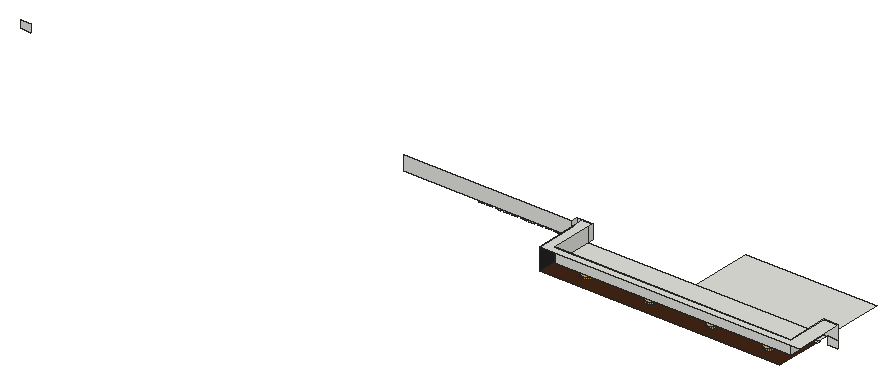
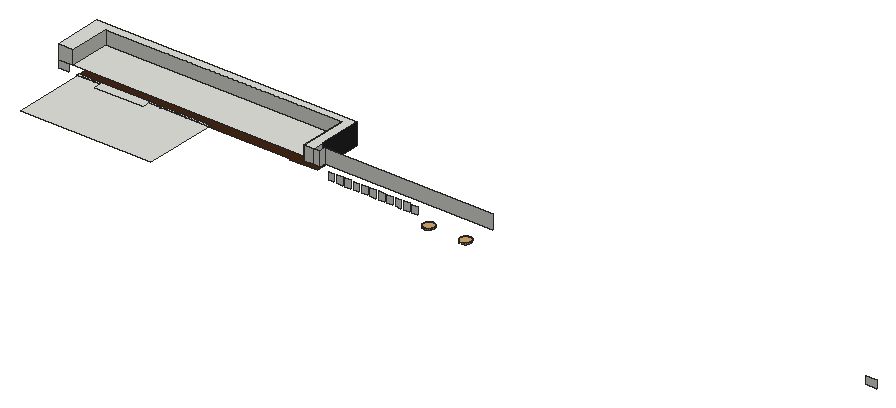
# SketchUp Ruby script. Lengths in inches.
U = 1.inch
M = Sketchup.active_model
def pt(a) = Geom::Point3d.new(a.map { |v| v * U })
def face(e, loops, mat)
  f = e.add_face(loops[0].map { |a| pt(a) })
  loops[1..].each { |l| e.add_face(l.map { |a| pt(a) }).erase! }
  f.material = f.back_material = mat if mat
  f
end
# faces: each face lists its corners as indices into pts; further lists are holes
def faces(e, pts, list, mat = nil) = list.each { |f| face(e, (f[0].is_a?(Array) ? f : [f]).map { |l| l.map { |i| pts[i] } }, mat) }
# xy, xz, yz: faces in a plane at the given z, y or x. An outline is a flat list of corners, or four numbers for a rectangle; further outlines are holes
def ring(l) = l.size == 4 ? [[l[0], l[1]], [l[2], l[1]], [l[2], l[3]], [l[0], l[3]]] : l.each_slice(2).to_a
def flat(e, list, mat, &to3) = list.each { |f| face(e, (f[0].is_a?(Array) ? f : [f]).map { |l| ring(l).map { |u, v| to3.(u, v) } }, mat) }
def xy(e, z, list, mat = nil) = flat(e, list, mat) { |x, y| [x, y, z] }
def xz(e, y, list, mat = nil) = flat(e, list, mat) { |x, z| [x, y, z] }
def yz(e, x, list, mat = nil) = flat(e, list, mat) { |y, z| [x, y, z] }
def lines(e, pts, list) = list.each { |a, b| e.add_line(pt(pts[a]), pt(pts[b])) }
# prism: a flat outline (further loops are holes) pulled along v
def prism(e, loops, v, mat = nil)
  f = face(e, loops, mat); d = Geom::Vector3d.new(v.map { |x| x * U })
  f.pushpull(f.normal.samedirection?(d) ? d.length : -d.length)
end
def box(e, o, s, mat = nil) = prism(e, [[o, [o[0] + s[0], o[1], o[2]], [o[0] + s[0], o[1] + s[1], o[2]], [o[0], o[1] + s[1], o[2]]]], [0, 0, s[2]], mat)
def at(x, y, z, deg = 0) = Geom::Transformation.translation(pt([x, y, z])) * Geom::Transformation.rotation(ORIGIN, Z_AXIS, deg.degrees)
def axes(o, x, y, z) = Geom::Transformation.new([*x, 0, *y, 0, *z, 0, *pt(o).to_a, 1])
def part(name) = M.definitions.add(name)
# library, detail: a bought-in or finely detailed component or shape, given as its bounding box
def library(name, o, s) = part(name).tap { |d| box(d.entities, o, s) }
def detail(e, o, s) = box(e.add_group.entities, o, s)
def put(e, d, t, mat = nil) = e.add_instance(d, t).tap { |i| i.material = mat if mat }
def group(e, t, mat = nil) = e.add_group.tap { |g| g.transformation = t; g.material = mat if mat }.entities
root = M.entities
M.materials.add("[Field Square Tile]").color = [211, 167, 108]
M.materials.add("[Granite Dark Gray]").color = [38, 37, 37]
M.materials.add("[Wood Veneer 01]").color = [66, 38, 20]
xy(root,380.5,[[1413.21,2343.96,1418.63,2346.71],[1418.63,2343.96,1419.83,2346.71],[1419.83,2343.96,1425.26,2346.71],[1425.26,2343.96,1426.46,2346.71],[1426.46,2343.96,1431.88,2346.71],
  [1431.88,2343.96,1433.08,2346.71],[1433.08,2343.96,1438.51,2346.71],[1438.51,2343.96,1439.71,2346.71],[1439.71,2343.96,1445.13,2346.71],[1445.13,2343.96,1446.33,2346.71],
  [1446.33,2343.96,1451.76,2346.71],[1451.76,2343.96,1452.96,2346.71],[1452.96,2343.96,1458.38,2346.71],[1458.38,2343.96,1459.58,2346.71],[1459.58,2343.96,1465.01,2346.71],
  [1465.01,2343.96,1466.21,2346.71],[1466.21,2343.96,1471.63,2346.71],[1471.63,2343.96,1472.83,2346.71],[1472.83,2343.96,1478.26,2346.71],[1478.26,2343.96,1531.81,2354.27],
  [1531.81,2343.96,1537.23,2346.71],[1537.23,2343.96,1538.43,2346.71],[1538.43,2343.96,1543.86,2346.71],[1543.86,2343.96,1545.06,2346.71],[1545.06,2343.96,1550.48,2346.71],
  [1550.48,2343.96,1551.31,2346.71],[1551.31,2343.96,1555.29,2346.71],[1555.29,2343.96,1556.73,2346.71],[1413.21,2346.71,1413.21,2425.46,1555.29,2425.46,1555.29,2346.71,1531.81,2346.71,1531.81,2354.27,1478.26,2354.27,1478.26,2346.71]])
xy(root,380.5,[[[1293.73,2294.125,1293.73,2347.9,1323.53,2347.9,1323.53,2346.71,1413.21,2346.71,1413.21,2343.96,1555.29,2343.96,1555.29,2294.125],[1529.08,2306.32,1530.64,2306.53,1532.08,2307.13,1533.33,2308.08,1534.28,2309.32,1534.88,2310.77,1535.08,2312.32,1534.88,2313.88,1534.28,2315.32,1533.33,2316.57,1532.08,2317.52,1530.64,2318.12,1529.08,2318.32,1527.53,2318.12,1526.08,2317.52,1524.84,2316.57,1523.89,2315.32,1523.29,2313.88,1523.08,2312.32,1523.29,2310.77,1523.89,2309.32,1524.84,2308.08,1526.08,2307.13,1527.53,2306.53],[1400.43,2306.32,1401.98,2306.53,1403.43,2307.13,1404.67,2308.08,1405.63,2309.32,1406.23,2310.77,1406.43,2312.32,1406.23,2313.88,1405.63,2315.32,1404.67,2316.57,1403.43,2317.52,1401.98,2318.12,1400.43,2318.32,1398.88,2318.12,1397.43,2317.52,1396.1875,2316.57,1395.24,2315.32,1394.64,2313.88,1394.43,2312.32,1394.64,2310.77,1395.24,2309.32,1396.1875,2308.08,1397.43,2307.13,1398.88,2306.53],[1330.97,2306.32,1332.52,2306.53,1333.97,2307.13,1335.21,2308.08,1336.16,2309.32,1336.76,2310.77,1336.97,2312.32,1336.76,2313.88,1336.16,2315.32,1335.21,2316.57,1333.97,2317.52,1332.52,2318.12,1330.97,2318.32,1329.42,2318.12,1327.97,2317.52,1326.73,2316.57,1325.77,2315.32,1325.17,2313.88,1324.97,2312.32,1325.17,2310.77,1325.77,2309.32,1326.73,2308.08,1327.97,2307.13,1329.42,2306.53],[1467.71,2306.32,1469.26,2306.53,1470.71,2307.13,1471.95,2308.08,1472.91,2309.32,1473.51,2310.77,1473.71,2312.32,1473.51,2313.88,1472.91,2315.32,1471.95,2316.57,1470.71,2317.52,1469.26,2318.12,1467.71,2318.32,1466.16,2318.12,1464.71,2317.52,1463.47,2316.57,1462.51,2315.32,1461.91,2313.88,1461.71,2312.32,1461.91,2310.77,1462.51,2309.32,1463.47,2308.08,1464.71,2307.13,1466.16,2306.53]]],"[Wood Veneer 01]")
xy(root,381.8125,[[1330.97,2306.32,1329.42,2306.53,1327.97,2307.13,1326.73,2308.08,1325.77,2309.32,1325.17,2310.77,1324.97,2312.32,1325.17,2313.88,1325.77,2315.32,1326.73,2316.57,1327.97,2317.52,1329.42,2318.12,1330.97,2318.32,1332.52,2318.12,1333.97,2317.52,1335.21,2316.57,1336.16,2315.32,1336.76,2313.88,1336.97,2312.32,1336.76,2310.77,1336.16,2309.32,1335.21,2308.08,1333.97,2307.13,1332.52,2306.53],[1400.43,2306.32,1398.88,2306.53,1397.43,2307.13,1396.1875,2308.08,1395.24,2309.32,1394.64,2310.77,1394.43,2312.32,1394.64,2313.88,1395.24,2315.32,1396.1875,2316.57,1397.43,2317.52,1398.88,2318.12,1400.43,2318.32,1401.98,2318.12,1403.43,2317.52,1404.67,2316.57,1405.63,2315.32,1406.23,2313.88,1406.43,2312.32,1406.23,2310.77,1405.63,2309.32,1404.67,2308.08,1403.43,2307.13,1401.98,2306.53],[1467.71,2306.32,1466.16,2306.53,1464.71,2307.13,1463.47,2308.08,1462.51,2309.32,1461.91,2310.77,1461.71,2312.32,1461.91,2313.88,1462.51,2315.32,1463.47,2316.57,1464.71,2317.52,1466.16,2318.12,1467.71,2318.32,1469.26,2318.12,1470.71,2317.52,1471.95,2316.57,1472.91,2315.32,1473.51,2313.88,1473.71,2312.32,1473.51,2310.77,1472.91,2309.32,1471.95,2308.08,1470.71,2307.13,1469.26,2306.53],[1529.08,2306.32,1527.53,2306.53,1526.08,2307.13,1524.84,2308.08,1523.89,2309.32,1523.29,2310.77,1523.08,2312.32,1523.29,2313.88,1523.89,2315.32,1524.84,2316.57,1526.08,2317.52,1527.53,2318.12,1529.08,2318.32,1530.64,2318.12,1532.08,2317.52,1533.33,2316.57,1534.28,2315.32,1534.88,2313.88,1535.08,2312.32,1534.88,2310.77,1534.28,2309.32,1533.33,2308.08,1532.08,2307.13,1530.64,2306.53]],"[Field Square Tile]")
xy(root,381.875,[[1119.58,2359.13,1118.02,2359.16,1116.51,2359.6,1115.17,2360.41,1114.09,2361.54,1113.33,2362.91,1112.96,2364.4375,1112.99,2366,1113.43,2367.51,1114.24,2368.85,1115.37,2369.93,1116.74,2370.69,1118.26,2371.06,1119.83,2371.03,1121.33,2370.59,1122.67,2369.78,1123.76,2368.65,1124.51,2367.28,1124.89,2365.75,1124.85,2364.1875,1124.42,2362.68,1123.61,2361.34,1122.48,2360.26,1121.1,2359.51],[1159.33,2359.13,1157.77,2359.16,1156.26,2359.6,1154.92,2360.41,1153.84,2361.54,1153.08,2362.91,1152.71,2364.4375,1152.74,2366,1153.18,2367.51,1153.99,2368.85,1155.12,2369.93,1156.49,2370.69,1158.01,2371.06,1159.58,2371.03,1161.08,2370.59,1162.42,2369.78,1163.51,2368.65,1164.26,2367.28,1164.64,2365.75,1164.6,2364.1875,1164.17,2362.68,1163.36,2361.34,1162.23,2360.26,1160.85,2359.51]],"[Field Square Tile]")
xy(root,388.625,[[1304.4375,2301.68,1560.93,2346.71]])
xy(root,403.8125,[[1293.73,2294.125,1576.91,2294.125,1576.91,2346.71,1560.93,2346.71,1560.93,2301.68,1304.4375,2301.68,1304.4375,2353.05,1293.73,2353.05]])
xz(root,2301.68,[[1304.4375,388.625,1560.93,403.8125]])
xz(root,2346.49,[[1104.06,388.625,1287.38,403.8125]])
xz(root,2346.71,[[686.35,380.5,698.16,388.625],[1565.1,380.5,1576.91,388.625],[1560.93,388.625,1576.91,403.8125]])
xz(root,2353.05,[[1287.38,388.625,1293.73,403.8125],[1293.73,388.625,1304.4375,403.8125]])
xz(root,2355.06,[[1178.68,380.5,1184.93,388.625],[1187.81,380.5,1194.06,388.625],[1196.93,380.5,1203.18,388.625],[1206.06,380.5,1212.31,388.625],[1215.18,380.5,1221.43,388.625],
  [1224.31,380.5,1230.56,388.625],[1233.43,380.5,1239.68,388.625],[1242.56,380.5,1248.81,388.625],[1251.68,380.5,1257.93,388.625],[1260.81,380.5,1267.06,388.625],
  [1269.93,380.5,1276.18,388.625]])
yz(root,1287.38,[[2346.49,388.625,2353.05,403.8125]])
yz(root,1293.73,[[2294.125,380.5,2340.15,403.8125]],"[Granite Dark Gray]")
yz(root,1304.4375,[[2301.68,388.625,2346.71,403.8125],[2346.71,388.625,2353.05,403.8125]])
yz(root,1560.93,[[2301.68,388.625,2346.71,403.8125]])
p = [[1330.97,2306.32,380.5],[1329.42,2306.53,380.5],[1329.42,2306.53,381.8125],[1330.97,2306.32,381.8125],[1332.52,2306.53,380.5],[1332.52,2306.53,381.8125],
  [1400.43,2306.32,380.5],[1398.88,2306.53,380.5],[1398.88,2306.53,381.8125],[1400.43,2306.32,381.8125],[1401.98,2306.53,380.5],[1401.98,2306.53,381.8125],
  [1467.71,2306.32,380.5],[1466.16,2306.53,380.5],[1466.16,2306.53,381.8125],[1467.71,2306.32,381.8125],[1469.26,2306.53,380.5],[1469.26,2306.53,381.8125],
  [1529.08,2306.32,380.5],[1527.53,2306.53,380.5],[1527.53,2306.53,381.8125],[1529.08,2306.32,381.8125],[1530.64,2306.53,380.5],[1530.64,2306.53,381.8125],
  [1327.97,2307.13,380.5],[1327.97,2307.13,381.8125],[1333.97,2307.13,380.5],[1333.97,2307.13,381.8125],[1397.43,2307.13,380.5],[1397.43,2307.13,381.8125],
  [1403.43,2307.13,380.5],[1403.43,2307.13,381.8125],[1464.71,2307.13,380.5],[1464.71,2307.13,381.8125],[1470.71,2307.13,380.5],[1470.71,2307.13,381.8125],
  [1526.08,2307.13,380.5],[1526.08,2307.13,381.8125],[1532.08,2307.13,380.5],[1532.08,2307.13,381.8125],[1326.73,2308.08,380.5],[1326.73,2308.08,381.8125],
  [1335.21,2308.08,380.5],[1335.21,2308.08,381.8125],[1396.1875,2308.08,380.5],[1396.1875,2308.08,381.8125],[1404.67,2308.08,380.5],[1404.67,2308.08,381.8125],
  [1463.47,2308.08,380.5],[1463.47,2308.08,381.8125],[1471.95,2308.08,380.5],[1471.95,2308.08,381.8125],[1524.84,2308.08,380.5],[1524.84,2308.08,381.8125],
  [1533.33,2308.08,380.5],[1533.33,2308.08,381.8125],[1325.77,2309.32,380.5],[1325.77,2309.32,381.8125],[1336.16,2309.32,380.5],[1336.16,2309.32,381.8125],
  [1395.24,2309.32,380.5],[1395.24,2309.32,381.8125],[1405.63,2309.32,380.5],[1405.63,2309.32,381.8125],[1462.51,2309.32,380.5],[1462.51,2309.32,381.8125],
  [1472.91,2309.32,380.5],[1472.91,2309.32,381.8125],[1523.89,2309.32,380.5],[1523.89,2309.32,381.8125],[1534.28,2309.32,380.5],[1534.28,2309.32,381.8125],
  [1325.17,2310.77,380.5],[1325.17,2310.77,381.8125],[1336.76,2310.77,380.5],[1336.76,2310.77,381.8125],[1394.64,2310.77,380.5],[1394.64,2310.77,381.8125],
  [1406.23,2310.77,380.5],[1406.23,2310.77,381.8125],[1461.91,2310.77,380.5],[1461.91,2310.77,381.8125],[1473.51,2310.77,380.5],[1473.51,2310.77,381.8125],
  [1523.29,2310.77,380.5],[1523.29,2310.77,381.8125],[1534.88,2310.77,380.5],[1534.88,2310.77,381.8125],[1324.97,2312.32,380.5],[1324.97,2312.32,381.8125],
  [1336.97,2312.32,380.5],[1336.97,2312.32,381.8125],[1394.43,2312.32,380.5],[1394.43,2312.32,381.8125],[1406.43,2312.32,380.5],[1406.43,2312.32,381.8125],
  [1461.71,2312.32,380.5],[1461.71,2312.32,381.8125],[1473.71,2312.32,380.5],[1473.71,2312.32,381.8125],[1523.08,2312.32,380.5],[1523.08,2312.32,381.8125],
  [1535.08,2312.32,380.5],[1535.08,2312.32,381.8125],[1325.17,2313.88,380.5],[1325.17,2313.88,381.8125],[1336.76,2313.88,380.5],[1336.76,2313.88,381.8125],
  [1394.64,2313.88,380.5],[1394.64,2313.88,381.8125],[1406.23,2313.88,380.5],[1406.23,2313.88,381.8125],[1461.91,2313.88,380.5],[1461.91,2313.88,381.8125],
  [1473.51,2313.88,380.5],[1473.51,2313.88,381.8125],[1523.29,2313.88,380.5],[1523.29,2313.88,381.8125],[1534.88,2313.88,380.5],[1534.88,2313.88,381.8125],
  [1325.77,2315.32,380.5],[1325.77,2315.32,381.8125],[1336.16,2315.32,380.5],[1336.16,2315.32,381.8125],[1395.24,2315.32,380.5],[1395.24,2315.32,381.8125],
  [1405.63,2315.32,380.5],[1405.63,2315.32,381.8125],[1462.51,2315.32,380.5],[1462.51,2315.32,381.8125],[1472.91,2315.32,380.5],[1472.91,2315.32,381.8125],
  [1523.89,2315.32,380.5],[1523.89,2315.32,381.8125],[1534.28,2315.32,380.5],[1534.28,2315.32,381.8125],[1326.73,2316.57,380.5],[1326.73,2316.57,381.8125],
  [1335.21,2316.57,380.5],[1335.21,2316.57,381.8125],[1396.1875,2316.57,380.5],[1396.1875,2316.57,381.8125],[1404.67,2316.57,380.5],[1404.67,2316.57,381.8125],
  [1463.47,2316.57,380.5],[1463.47,2316.57,381.8125],[1471.95,2316.57,380.5],[1471.95,2316.57,381.8125],[1524.84,2316.57,380.5],[1524.84,2316.57,381.8125],
  [1533.33,2316.57,380.5],[1533.33,2316.57,381.8125],[1327.97,2317.52,380.5],[1327.97,2317.52,381.8125],[1333.97,2317.52,380.5],[1333.97,2317.52,381.8125],
  [1397.43,2317.52,380.5],[1397.43,2317.52,381.8125],[1403.43,2317.52,380.5],[1403.43,2317.52,381.8125],[1464.71,2317.52,380.5],[1464.71,2317.52,381.8125],
  [1470.71,2317.52,380.5],[1470.71,2317.52,381.8125],[1526.08,2317.52,380.5],[1526.08,2317.52,381.8125],[1532.08,2317.52,380.5],[1532.08,2317.52,381.8125],
  [1329.42,2318.12,380.5],[1329.42,2318.12,381.8125],[1332.52,2318.12,380.5],[1332.52,2318.12,381.8125],[1398.88,2318.12,380.5],[1398.88,2318.12,381.8125],
  [1401.98,2318.12,380.5],[1401.98,2318.12,381.8125],[1466.16,2318.12,380.5],[1466.16,2318.12,381.8125],[1469.26,2318.12,380.5],[1469.26,2318.12,381.8125],
  [1527.53,2318.12,380.5],[1527.53,2318.12,381.8125],[1530.64,2318.12,380.5],[1530.64,2318.12,381.8125],[1330.97,2318.32,380.5],[1330.97,2318.32,381.8125],
  [1400.43,2318.32,380.5],[1400.43,2318.32,381.8125],[1467.71,2318.32,380.5],[1467.71,2318.32,381.8125],[1529.08,2318.32,380.5],[1529.08,2318.32,381.8125],
  [1119.58,2359.13,380.5],[1118.02,2359.16,380.5],[1118.02,2359.16,381.875],[1119.58,2359.13,381.875],[1121.1,2359.51,380.5],[1121.1,2359.51,381.875],
  [1159.33,2359.13,380.5],[1157.77,2359.16,380.5],[1157.77,2359.16,381.875],[1159.33,2359.13,381.875],[1160.85,2359.51,380.5],[1160.85,2359.51,381.875],
  [1116.51,2359.6,380.5],[1116.51,2359.6,381.875],[1156.26,2359.6,380.5],[1156.26,2359.6,381.875],[1122.48,2360.26,380.5],[1122.48,2360.26,381.875],
  [1162.23,2360.26,380.5],[1162.23,2360.26,381.875],[1115.17,2360.41,380.5],[1115.17,2360.41,381.875],[1154.92,2360.41,380.5],[1154.92,2360.41,381.875],
  [1123.61,2361.34,380.5],[1123.61,2361.34,381.875],[1163.36,2361.34,380.5],[1163.36,2361.34,381.875],[1114.09,2361.54,380.5],[1114.09,2361.54,381.875],
  [1153.84,2361.54,380.5],[1153.84,2361.54,381.875],[1124.42,2362.68,380.5],[1124.42,2362.68,381.875],[1164.17,2362.68,380.5],[1164.17,2362.68,381.875],
  [1113.33,2362.91,380.5],[1113.33,2362.91,381.875],[1153.08,2362.91,380.5],[1153.08,2362.91,381.875],[1124.85,2364.1875,380.5],[1124.85,2364.1875,381.875],
  [1164.6,2364.1875,380.5],[1164.6,2364.1875,381.875],[1112.96,2364.4375,380.5],[1112.96,2364.4375,381.875],[1152.71,2364.4375,380.5],[1152.71,2364.4375,381.875],
  [1124.89,2365.75,380.5],[1124.89,2365.75,381.875],[1164.64,2365.75,380.5],[1164.64,2365.75,381.875],[1112.99,2366,380.5],[1112.99,2366,381.875],
  [1152.74,2366,380.5],[1152.74,2366,381.875],[1124.51,2367.28,380.5],[1124.51,2367.28,381.875],[1164.26,2367.28,380.5],[1164.26,2367.28,381.875],
  [1113.43,2367.51,380.5],[1113.43,2367.51,381.875],[1153.18,2367.51,380.5],[1153.18,2367.51,381.875],[1123.76,2368.65,380.5],[1123.76,2368.65,381.875],
  [1163.51,2368.65,380.5],[1163.51,2368.65,381.875],[1114.24,2368.85,380.5],[1114.24,2368.85,381.875],[1153.99,2368.85,380.5],[1153.99,2368.85,381.875],
  [1122.67,2369.78,380.5],[1122.67,2369.78,381.875],[1162.42,2369.78,380.5],[1162.42,2369.78,381.875],[1115.37,2369.93,380.5],[1115.37,2369.93,381.875],
  [1155.12,2369.93,380.5],[1155.12,2369.93,381.875],[1121.33,2370.59,380.5],[1121.33,2370.59,381.875],[1161.08,2370.59,380.5],[1161.08,2370.59,381.875],
  [1116.74,2370.69,380.5],[1116.74,2370.69,381.875],[1156.49,2370.69,380.5],[1156.49,2370.69,381.875],[1119.83,2371.03,380.5],[1119.83,2371.03,381.875],
  [1159.58,2371.03,380.5],[1159.58,2371.03,381.875],[1118.26,2371.06,380.5],[1118.26,2371.06,381.875],[1158.01,2371.06,380.5],[1158.01,2371.06,381.875],
  [1293.75,2303.93,380.5],[1293.73,2294.125,380.5]]
faces(root,p,[[0,1,2,3],[4,0,3,5],[6,7,8,9],[10,6,9,11],[12,13,14,15],[16,12,15,17],[18,19,20,21],[22,18,21,23],
  [1,24,25,2],[26,4,5,27],[7,28,29,8],[30,10,11,31],[13,32,33,14],[34,16,17,35],[19,36,37,20],[38,22,23,39],
  [24,40,41,25],[42,26,27,43],[28,44,45,29],[46,30,31,47],[32,48,49,33],[50,34,35,51],[36,52,53,37],[54,38,39,55],
  [40,56,57,41],[58,42,43,59],[44,60,61,45],[62,46,47,63],[48,64,65,49],[66,50,51,67],[52,68,69,53],[70,54,55,71],
  [56,72,73,57],[74,58,59,75],[60,76,77,61],[78,62,63,79],[64,80,81,65],[82,66,67,83],[68,84,85,69],[86,70,71,87],
  [72,88,89,73],[90,74,75,91],[76,92,93,77],[94,78,79,95],[80,96,97,81],[98,82,83,99],[84,100,101,85],[102,86,87,103],
  [88,104,105,89],[106,90,91,107],[92,108,109,93],[110,94,95,111],[96,112,113,97],[114,98,99,115],[100,116,117,101],[118,102,103,119],
  [104,120,121,105],[122,106,107,123],[108,124,125,109],[126,110,111,127],[112,128,129,113],[130,114,115,131],[116,132,133,117],[134,118,119,135],
  [120,136,137,121],[138,122,123,139],[124,140,141,125],[142,126,127,143],[128,144,145,129],[146,130,131,147],[132,148,149,133],[150,134,135,151],
  [136,152,153,137],[154,138,139,155],[140,156,157,141],[158,142,143,159],[144,160,161,145],[162,146,147,163],[148,164,165,149],[166,150,151,167],
  [152,168,169,153],[170,154,155,171],[156,172,173,157],[174,158,159,175],[160,176,177,161],[178,162,163,179],[164,180,181,165],[182,166,167,183],
  [168,184,185,169],[184,170,171,185],[172,186,187,173],[186,174,175,187],[176,188,189,177],[188,178,179,189],[180,190,191,181],[190,182,183,191],
  [192,193,194,195],[196,192,195,197],[198,199,200,201],[202,198,201,203],[193,204,205,194],[199,206,207,200],[208,196,197,209],[210,202,203,211],
  [204,212,213,205],[206,214,215,207],[216,208,209,217],[218,210,211,219],[212,220,221,213],[214,222,223,215],[224,216,217,225],[226,218,219,227],
  [220,228,229,221],[222,230,231,223],[232,224,225,233],[234,226,227,235],[228,236,237,229],[230,238,239,231],[240,232,233,241],[242,234,235,243],
  [236,244,245,237],[238,246,247,239],[248,240,241,249],[250,242,243,251],[244,252,253,245],[246,254,255,247],[256,248,249,257],[258,250,251,259],
  [252,260,261,253],[254,262,263,255],[264,256,257,265],[266,258,259,267],[260,268,269,261],[262,270,271,263],[272,264,265,273],[274,266,267,275],
  [268,276,277,269],[270,278,279,271],[280,272,273,281],[282,274,275,283],[276,284,285,277],[278,286,287,279]],"[Field Square Tile]")
lines(root,p,[[288,289]])
